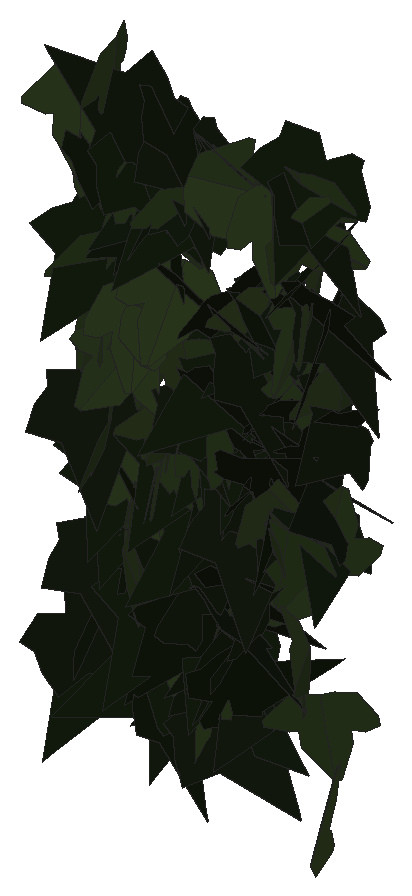
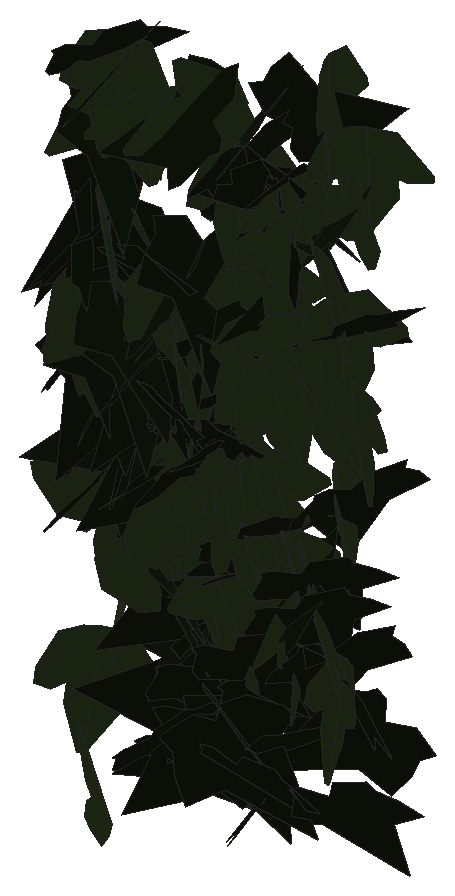
# SketchUp Ruby script. Lengths in inches.
U = 1.inch
M = Sketchup.active_model
def pt(a) = Geom::Point3d.new(a.map { |v| v * U })
def face(e, loops, mat)
  f = e.add_face(loops[0].map { |a| pt(a) })
  loops[1..].each { |l| e.add_face(l.map { |a| pt(a) }).erase! }
  f.material = f.back_material = mat if mat
  f
end
# faces: each face lists its corners as indices into pts; further lists are holes
def faces(e, pts, list, mat = nil) = list.each { |f| face(e, (f[0].is_a?(Array) ? f : [f]).map { |l| l.map { |i| pts[i] } }, mat) }
# xy, xz, yz: faces in a plane at the given z, y or x. An outline is a flat list of corners, or four numbers for a rectangle; further outlines are holes
def ring(l) = l.size == 4 ? [[l[0], l[1]], [l[2], l[1]], [l[2], l[3]], [l[0], l[3]]] : l.each_slice(2).to_a
def flat(e, list, mat, &to3) = list.each { |f| face(e, (f[0].is_a?(Array) ? f : [f]).map { |l| ring(l).map { |u, v| to3.(u, v) } }, mat) }
def xy(e, z, list, mat = nil) = flat(e, list, mat) { |x, y| [x, y, z] }
def xz(e, y, list, mat = nil) = flat(e, list, mat) { |x, z| [x, y, z] }
def yz(e, x, list, mat = nil) = flat(e, list, mat) { |y, z| [x, y, z] }
def lines(e, pts, list) = list.each { |a, b| e.add_line(pt(pts[a]), pt(pts[b])) }
# prism: a flat outline (further loops are holes) pulled along v
def prism(e, loops, v, mat = nil)
  f = face(e, loops, mat); d = Geom::Vector3d.new(v.map { |x| x * U })
  f.pushpull(f.normal.samedirection?(d) ? d.length : -d.length)
end
def box(e, o, s, mat = nil) = prism(e, [[o, [o[0] + s[0], o[1], o[2]], [o[0] + s[0], o[1] + s[1], o[2]], [o[0], o[1] + s[1], o[2]]]], [0, 0, s[2]], mat)
def at(x, y, z, deg = 0) = Geom::Transformation.translation(pt([x, y, z])) * Geom::Transformation.rotation(ORIGIN, Z_AXIS, deg.degrees)
def axes(o, x, y, z) = Geom::Transformation.new([*x, 0, *y, 0, *z, 0, *pt(o).to_a, 1])
def part(name) = M.definitions.add(name)
# library, detail: a bought-in or finely detailed component or shape, given as its bounding box
def library(name, o, s) = part(name).tap { |d| box(d.entities, o, s) }
def detail(e, o, s) = box(e.add_group.entities, o, s)
def put(e, d, t, mat = nil) = e.add_instance(d, t).tap { |i| i.material = mat if mat }
def group(e, t, mat = nil) = e.add_group.tap { |g| g.transformation = t; g.material = mat if mat }.entities
root = M.entities
M.materials.add("efeu1").color = [18, 25, 13]
M.materials.add("efeu2").color = [43, 57, 29]
c1 = part("ivyleaf_9")
p = [[1.54,2.16,1.25],[1.36,2.04,1.19],[-0.21,0.99,0.68],[-0.71,1.11,0.82],[-0.85,0.86,0.67],[-0.8,0.17,0.21],
  [-0.9,-0.01,0.1],[-0.67,-0.16,-0.02],[-0.08,-0.08,-0.05],[-0.03,-0.6,-0.4],[0.65,-0.88,-0.66],[0.83,-0.6,-0.49],
  [1.29,-0.42,-0.43],[1.8125,-0.07,-0.26],[1.21,0.44,0.15]]
faces(c1.entities,p,[[0,1,2,3,4,5,6,7,8,9,10,11,12,13,14]],"efeu1")
c2 = part("ivyleaf_10")
p = [[0,0.5,-0.03],[-0.0625,2.02,-0.43],[-0.19,2.01,-0.46],[-0.54,1.05,-0.29],[-0.52,0.625,-0.18],[-0.83,0.76,-0.28],
  [-1.16,0.64,-0.33],[-1.15,0.33,-0.24],[-0.77,-0.39,0.02],[-0.3,-0.51,0.16],[0.04,-0.48,0.23],[-0.02,2.01,-0.4375],
  [-0.06,2.01,-0.43],[0.04,-0.49,0.23],[0.67,-0.49,0.14],[1.38,0.36,-0.2],[1.375,0.51,-0.24],[0.81,0.65,-0.19],
  [0.62,0.59,-0.15],[0.6,1.09,-0.28],[0.5,1.23,-0.31]]
faces(c2.entities,p,[[0,1,2,3,4,5,6,7,8,9,10],[11,12,0,13,14,15,16,17,18,19,20]],"efeu2")
put(root,c1,axes([43.54,222.53,237.25],[0.46224,0.15127,-0.116],[0.11056,0.0351,0.48636],[0.15529,-0.47527,-0.00101]))
put(root,c1,axes([44.33,222.78,241.43],[-0.26887,-0.42118,0.01772],[0.03089,-0.04064,-0.49739],[0.42042,-0.26637,0.04787]))
put(root,c1,axes([41.21,222.68,237.46],[-0.08597,-0.48303,-0.09641],[0.03491,0.09165,-0.49029],[0.49131,-0.09104,0.01797]))
put(root,c1,axes([43.4,222.62,238.74],[0.20242,-0.4554,-0.0405],[-0.01543,0.03746,-0.49836],[0.45693,0.20301,0.00111]))
put(root,c2,axes([41.53,222.4375,237.27],[0.17347,-0.43056,-0.18582],[-0.06305,0.17491,-0.46415],[0.46469,0.18446,0.00639]))
put(root,c1,axes([42.93,222.35,235.55],[-0.116,0.12484,0.47006],[-0.34623,0.31818,-0.16994],[-0.34156,-0.36493,0.01263]))
put(root,c1,axes([42.04,222.5,241.2],[-0.05864,0.03305,0.49545],[-0.45265,0.20154,-0.06702],[-0.20414,-0.45639,0.00628]))
put(root,c2,axes([41.1,222.62,241.3],[-0.45326,-0.21028,0.0183],[0.06607,-0.18252,-0.46078],[0.20047,-0.4153,0.19324]))
put(root,c2,axes([41.92,222.54,238.97],[0.36604,0.3394,-0.02879],[-0.02117,-0.01951,-0.49917],[-0.33996,0.36665,0.00008]))
put(root,c2,axes([44.09,222.59,239.52],[0.39246,-0.30886,-0.02416],[-0.01952,0.01427,-0.49942],[0.30918,0.39294,-0.00086]))
put(root,c1,axes([42.7,222.65,235.28],[0.06829,0.23595,-0.43551],[-0.10368,-0.42308,-0.24547],[-0.48434,0.12384,-0.00886]))
put(root,c1,axes([43.36,222.73,236.66],[-0.10242,-0.48425,-0.07077],[0.02536,0.06696,-0.49485],[0.48874,-0.10495,0.01084]))
put(root,c1,axes([42.11,222.46,240.21],[-0.36634,0.33812,0.03838],[-0.0259,0.02852,-0.49851],[-0.3393,-0.36724,-0.00339]))
put(root,c2,axes([44,222.83,235.11],[-0.14747,0.00715,0.4777],[0.3485,-0.34037,0.11268],[0.32681,0.36619,0.09541]))
put(root,c1,axes([42.43,222.63,239.28],[0.27758,-0.26965,0.31661],[0.29438,-0.14148,-0.37859],[0.29376,0.39658,0.08022]))
put(root,c1,axes([44.24,222.6,241.11],[0.23225,-0.43216,-0.09644],[-0.01298,0.10221,-0.48927],[0.4426,0.22977,0.03625]))
put(root,c2,axes([41.75,222.55,238.27],[0.42519,0.0263,-0.26177],[-0.26303,0.05257,-0.42196],[0.00533,0.49653,0.05854]))
put(root,c2,axes([44.39,222.31,240.8125],[-0.19601,-0.26063,-0.37901],[0.24554,0.28909,-0.32578],[0.38896,-0.31384,0.01467]))
put(root,c2,axes([42.41,222.6,239.36],[0.41704,0.24252,-0.13138],[-0.12281,-0.04998,-0.4821],[-0.24697,0.43438,0.01788]))
put(root,c1,axes([42.53,222.83,240.49],[-0.38364,-0.30971,0.08308],[-0.06938,-0.04631,-0.49299],[0.31306,-0.38979,-0.00744]))
put(root,c1,axes([42.48,222.67,240.68],[-0.49563,0.05348,0.03861],[-0.03939,-0.0052,-0.49842],[-0.05291,-0.4971,0.00937]))
put(root,c1,axes([42.11,222.9,234.29],[-0.37796,-0.1692,0.28022],[-0.19084,-0.23386,-0.39861],[0.26595,-0.40827,0.1122]))
put(root,c1,axes([41.08,222.41,234.77],[0.07274,-0.12619,-0.47831],[0.24955,0.42679,-0.07464],[0.42712,-0.22787,0.12507]))
put(root,c1,axes([41.24,222.47,240.75],[0.37142,-0.27383,-0.19253],[-0.11361,0.16739,-0.45725],[0.31487,0.38341,0.06212]))
put(root,c2,axes([43.79,222.56,240.81],[0.25572,0.42952,-0.01094],[-0.00033,-0.01254,-0.49984],[-0.42966,0.25565,-0.00612]))
put(root,c2,axes([42.67,222.55,240.52],[-0.30459,-0.39138,-0.06357],[0.04452,0.04589,-0.49589],[0.39401,-0.30775,0.00689]))
put(root,c1,axes([41.21,222.94,239.34],[-0.28961,-0.38438,0.13557],[0.00723,-0.17112,-0.46975],[0.40752,-0.27013,0.10467]))
put(root,c2,axes([44.03,222.56,236.66],[-0.46662,-0.11221,0.14027],[-0.13807,-0.02574,-0.47987],[0.11492,-0.48657,-0.00697]))
put(root,c2,axes([41.53,222.58,241.92],[0.12375,-0.4795,-0.06904],[0.0585,0.08553,-0.48914],[0.4809,0.11299,0.07727]))
put(root,c2,axes([41.09,222.72,240.63],[0.22306,-0.06731,0.4424],[0.43464,-0.08499,-0.23208],[0.10644,0.4881,0.02059]))
put(root,c1,axes([42.25,222.77,241.34],[0.2103,-0.44999,0.05732],[0.0192,-0.0543,-0.49667],[0.45322,0.2111,-0.00556]))
put(root,c1,axes([43.06,222.78,237.04],[-0.45318,0.0002,-0.21125],[0.20958,-0.06218,-0.44968],[-0.02646,-0.49612,0.05628]))
put(root,c1,axes([42.84,222.71,237.83],[0.17704,-0.14553,0.44438],[0.36361,-0.25593,-0.22867],[0.29402,0.40413,0.01521]))
put(root,c1,axes([43.07,222.69,235.41],[0.32484,-0.3525,0.14222],[0.15011,-0.0529,-0.47399],[0.34921,0.35064,0.07146]))
put(root,c1,axes([41.84,222.59,240.82],[0.18669,-0.4129,-0.21134],[0.01255,0.23223,-0.44262],[0.46367,0.15996,0.09707]))
put(root,c2,axes([44.24,222.5625,241.21],[-0.49734,-0.05058,0.00982],[-0.01012,0.00247,-0.49989],[0.05052,-0.49743,-0.00349]))
put(root,c1,axes([41.35,222.76,235.65],[-0.09243,-0.45518,-0.18513],[0.06497,0.1754,-0.4637],[0.48707,-0.10978,0.02672]))
put(root,c1,axes([43.11,222.89,238.35],[-0.45024,-0.18225,0.11861],[-0.11115,-0.04152,-0.48572],[0.18689,-0.46375,-0.00313]))
put(root,c1,axes([44.48,222.375,240.3125],[-0.08007,0.47021,0.14998],[-0.06984,0.13962,-0.475],[-0.48858,-0.09701,0.04332]))
put(root,c1,axes([42.11,222.95,235.14],[-0.32486,-0.37401,0.0677],[-0.04828,-0.04773,-0.49537],[0.37701,-0.32839,-0.00511]))
put(root,c2,axes([41.95,222.61,240.55],[0.06822,0.49532,0.0024],[-0.00265,0.00279,-0.49999],[-0.49532,0.06821,0.00301]))
put(root,c2,axes([43.09,222.375,240.93],[0.11835,0.09672,0.47606],[0.23167,0.41944,-0.14282],[-0.42699,0.25438,0.05447]))
put(root,c1,axes([44.29,223.07,237.1],[-0.05895,-0.18464,0.46091],[-0.05296,-0.45916,-0.19071],[0.49368,-0.0713,0.03458]))
put(root,c2,axes([42.57,222.77,234.35],[0.4838,-0.09505,0.08308],[0.08028,-0.02229,-0.49301],[0.09743,0.49038,-0.00631]))
put(root,c1,axes([43.01,222.48,235.76],[0.46479,0.09077,0.16041],[0.1566,0.03504,-0.47355],[-0.09721,0.49044,0.00414]))
put(root,c1,axes([43.17,222.7,235.24],[-0.4087,0.28596,-0.03458],[0.03373,-0.0121,-0.49871],[-0.28606,-0.40998,-0.0094]))
put(root,c2,axes([41.88,222.5,235.68],[-0.2152,0.38535,0.23494],[-0.15893,0.1789,-0.43902],[-0.42241,-0.26363,0.04549]))
put(root,c1,axes([42.05,222.83,233.95],[0.23568,-0.44035,-0.02338],[-0.01161,0.02031,-0.49945],[0.44082,0.23597,-0.00065]))
put(root,c2,axes([43.89,222.55,237.2],[-0.21134,-0.35607,-0.28026],[0.14901,0.23744,-0.41403],[0.42794,-0.25852,0.00575]))
put(root,c1,axes([41.16,222.9,235.44],[-0.36905,-0.02771,-0.33621],[0.33735,-0.03036,-0.3678],[-0.00004,-0.49831,0.0411]))
put(root,c1,axes([42.37,222.875,241.01],[0.05277,-0.48849,-0.09269],[-0.01564,0.09153,-0.4913],[0.49696,0.05475,-0.00562]))
put(root,c1,axes([42.65,223.11,236.08],[-0.37114,-0.26984,0.1986],[-0.04136,-0.25721,-0.42677],[0.33249,-0.33321,0.1686]))
put(root,c1,axes([44.39,223.14,238.08],[-0.08884,-0.31186,0.38059],[-0.03628,-0.38154,-0.32111],[0.4907,-0.08467,0.04516]))
put(root,c1,axes([43.69,222.59,235.79],[-0.30283,0.36432,0.15988],[-0.11252,0.11429,-0.47358],[-0.38162,-0.32281,0.01276]))
put(root,c2,axes([42.15,222.46,238.94],[0.15593,0.16079,0.44703],[0.22157,0.39157,-0.21813],[-0.42023,0.26612,0.05087]))
put(root,c2,axes([42.5,222.71,238.44],[-0.4486,-0.21904,-0.02789],[0.02371,0.01499,-0.49921],[0.21953,-0.44922,-0.00306]))
put(root,c2,axes([43.61,222.59,236.78],[-0.36045,0.1622,0.30621],[-0.28549,0.1114,-0.39507],[-0.19639,-0.45965,0.01231]))
put(root,c2,axes([41.28,222.77,239.375],[-0.18752,-0.46324,-0.0158],[-0.0017,0.01773,-0.49968],[0.4635,-0.18734,-0.00822]))
put(root,c2,axes([42.05,222.91,238.5],[-0.13518,-0.45783,0.14871],[-0.02121,-0.14865,-0.47692],[0.48091,-0.13524,0.02077]))
put(root,c2,axes([41.48,222.8,239.94],[0.37888,-0.31492,-0.0853],[-0.05638,0.06556,-0.49247],[0.32136,0.38279,0.01417]))
put(root,c1,axes([42.95,222.77,241.05],[0.41235,-0.2487,0.13461],[0.15086,-0.00785,-0.47663],[0.23919,0.43369,0.06856]))
put(root,c1,axes([41.9,222.93,240.36],[-0.12662,-0.0082,-0.48363],[0.48362,0.00724,-0.12674],[0.00908,-0.49988,0.0061]))
put(root,c1,axes([44.03,222.625,239.7],[0.49536,0.04115,0.05411],[0.05474,-0.00553,-0.49696],[-0.0403,0.49827,-0.00998]))
put(root,c2,axes([41.8125,222.875,236.68],[0.38641,-0.31726,0.00575],[0.00385,-0.00438,-0.49997],[0.31728,0.38643,-0.00094]))
put(root,c2,axes([42.19,222.8125,237.06],[-0.41634,0.1016,0.25756],[-0.27576,-0.1106,-0.40215],[-0.02474,-0.47691,0.14813]))
put(root,c2,axes([41.08,222.77,238.52],[0.4018,-0.27518,-0.11329],[-0.04383,0.13354,-0.47984],[0.29434,0.39553,0.08319]))
put(root,c1,axes([43.15,222.61,239.49],[-0.02074,0.49729,-0.04769],[0.01255,-0.0472,-0.49761],[-0.49941,-0.02184,-0.01052]))
put(root,c1,axes([41.16,223.03,234.17],[-0.42793,-0.25439,-0.04647],[0.0371,0.02852,-0.49781],[0.25592,-0.4295,-0.00553]))
put(root,c2,axes([41.76,222.89,236.61],[0.36146,-0.34541,0.00585],[-0.00138,-0.00991,-0.4999],[0.34546,0.36137,-0.00812]))
put(root,c1,axes([43.07,222.51,234.4],[0.16173,0.08903,0.46467],[0.41569,0.20777,-0.18449],[-0.22594,0.44599,-0.00681]))
put(root,c1,axes([43.04,223.03,237.63],[-0.36746,-0.30638,-0.14526],[0.13957,0.05853,-0.47654],[0.30901,-0.39077,0.04251]))
put(root,c2,axes([43.9,222.93,235.93],[-0.1448,0.08012,-0.47182],[-0.47458,-0.08756,0.13078],[-0.06167,0.48571,0.1014]))
put(root,c2,axes([44.33,222.79,234.6],[-0.41247,-0.27968,-0.04056],[0.03592,0.01929,-0.49833],[0.28031,-0.41401,0.00417]))
put(root,c2,axes([44.28,222.8,232.89],[0.32162,-0.37822,0.05926],[-0.03848,0.04507,0.49648],[-0.3809,-0.32391,-0.00012]))
put(root,c1,axes([43.63,223.125,237.17],[-0.07854,0.04571,-0.49167],[0.38472,-0.30643,-0.08994],[-0.30955,-0.39244,0.01296]))
put(root,c1,axes([42.7,222.86,234.59],[-0.43942,0.23839,0.00924],[-0.00679,0.00686,-0.49991],[-0.23847,-0.43946,-0.00279]))
put(root,c1,axes([42.5,222.96,237.71],[0.08377,-0.47898,-0.11644],[0.09221,0.13125,-0.47357],[0.48423,0.05787,0.11033]))
put(root,c1,axes([43.73,223,239.28],[-0.49983,-0.0111,0.00716],[-0.00729,0.00605,-0.49991],[0.01101,-0.49984,-0.00621]))
put(root,c1,axes([44.24,223.13,239.47],[-0.19198,0.02738,-0.46086],[0.38663,-0.26324,-0.1767],[-0.25231,-0.42421,0.07991]))
put(root,c2,axes([44.28,222.9,236.47],[-0.40174,-0.28743,0.07738],[0.06544,0.04151,0.49396],[-0.29038,0.40701,0.00427]))
put(root,c2,axes([42.6,222.86,237.44],[0.04224,0.49346,-0.06865],[-0.01449,-0.06764,-0.49519],[-0.498,0.04383,0.00859]))
put(root,c2,axes([41.75,222.83,236.68],[0.47502,0.07575,0.13643],[0.11641,0.1191,-0.47145],[-0.10392,0.47966,0.09552]))
put(root,c1,axes([44.08,223.22,236.74],[-0.01739,-0.46494,0.1831],[0.0375,-0.18391,-0.46343],[0.49829,-0.00239,0.04127]))
put(root,c1,axes([42.83,222.85,233.99],[-0.00501,-0.28078,-0.41369],[0.24937,0.35717,-0.24544],[0.43335,-0.20879,0.13646]))
put(root,c2,axes([43.33,223.03,239.23],[-0.13587,-0.46833,0.11047],[-0.00946,-0.11217,-0.48716],[0.48109,-0.13447,0.02162]))
put(root,c2,axes([43.02,222.8,237.59],[0.00825,0.49162,0.0908],[-0.02455,0.09111,-0.49102],[-0.49933,0.00364,0.02564]))
put(root,c1,axes([42.71,223.17,235.14],[-0.29693,-0.39696,-0.06523],[0.03959,0.05184,-0.49573],[0.40033,-0.29956,0.00065]))
put(root,c2,axes([43.06,222.93,236.89],[-0.45518,-0.07823,-0.19156],[0.20073,-0.05458,-0.45468],[0.05023,-0.49082,0.08109]))
put(root,c1,axes([42.11,223.29,236.9],[-0.29805,-0.38784,0.10365],[0.01238,-0.13791,-0.48045],[0.40126,-0.28383,0.09181]))
put(root,c2,axes([42.11,223.03,237.4],[-0.23117,-0.43348,0.09303],[-0.03948,-0.08437,-0.49125],[0.44159,-0.23447,0.00478]))
put(root,c2,axes([43.23,222.86,238.66],[-0.43433,0.21175,0.12852],[-0.13258,0.0204,-0.48167],[-0.20923,-0.45249,0.03842]))
put(root,c2,axes([42.54,223.05,235.54],[0.44209,-0.20977,0.10271],[0.10163,-0.02519,-0.48891],[0.2103,0.45317,0.02036]))
put(root,c1,axes([44.16,222.63,237.95],[0.19586,0.44313,0.12358],[0.06323,0.10711,-0.48428],[-0.45568,0.20533,-0.01408]))
put(root,c1,axes([43.22,223.03,239.13],[0.34758,-0.35737,0.03839],[0.06158,0.00659,-0.49615],[0.35411,0.34964,0.04859]))
put(root,c2,axes([44.03,223.03,239.75],[0.29733,-0.40189,-0.00863],[0.03524,0.03675,-0.4974],[0.40044,0.29518,0.05018]))
put(root,c2,axes([44.39,222.98,238.72],[-0.05699,-0.49233,-0.06607],[0.01266,0.06504,-0.49559],[0.49658,-0.05816,0.00505]))
put(root,c2,axes([41.28,223.11,236.2],[0.36967,-0.32472,0.08886],[0.06679,-0.05861,-0.49204],[0.32997,0.37566,0.00005]))
put(root,c1,axes([44.23,223.07,239.43],[0.16513,-0.45771,-0.11504],[-0.001,0.12154,-0.485],[0.47194,0.16041,0.03922]))
put(root,c1,axes([42.64,222.93,234.22],[0.06672,-0.2029,-0.45209],[0.32479,0.36242,-0.11472],[0.37424,-0.27836,0.18016]))
put(root,c1,axes([44.02,222.78,238.35],[0.09409,0.48324,-0.08731],[-0.06881,-0.07505,-0.48952],[-0.48622,0.10414,0.05239]))
put(root,c2,axes([42.22,223.02,237.41],[0.06589,-0.4939,-0.04144],[0.01246,0.04345,-0.49795],[0.49548,0.06459,0.01803]))
put(root,c1,axes([43.58,222.9,237.46],[0.44155,-0.16585,0.16591],[0.19303,0.05591,-0.45784],[0.13332,0.46837,0.1134]))
put(root,c1,axes([42.93,223.22,237.71],[-0.45632,-0.20192,-0.03163],[0.02986,0.01068,-0.49899],[0.20218,-0.45729,0.00231]))
put(root,c1,axes([41.33,223.27,236.73],[-0.32225,-0.38019,-0.04017],[0.0591,0.00237,-0.49649],[0.37771,-0.32474,0.04341]))
put(root,c1,axes([43.36,223.15,238.4],[0.1694,-0.46954,-0.02898],[0.00779,0.0336,-0.49881],[0.47036,0.16855,0.0187]))
put(root,c1,axes([42.78,223.22,237.48],[0.00666,-0.49913,-0.02866],[0.01569,0.02885,-0.49892],[0.49971,0.00574,0.01605]))
put(root,c2,axes([43.11,223.34,236.84],[-0.21403,-0.26133,0.36864],[0.02211,-0.41347,-0.28027],[0.45133,-0.10367,0.18855]))
put(root,c2,axes([41.66,222.99,240.47],[0.04416,0.49717,-0.02958],[-0.00834,-0.02895,-0.49909],[-0.49798,0.04457,0.00574]))
put(root,c1,axes([42.51,223.125,234.56],[0.0416,0.17873,-0.46511],[-0.27166,-0.38312,-0.17152],[-0.4177,0.26697,0.06523]))
put(root,c2,axes([41.19,222.9375,235.42],[-0.42153,0.24684,0.1067],[-0.10347,0.03425,-0.48798],[-0.24821,-0.43347,0.02221]))
put(root,c1,axes([42.17,223.25,234.27],[-0.42098,-0.18976,-0.19174],[0.1982,0.0235,-0.45844],[0.183,-0.46199,0.05543]))
put(root,c1,axes([41.4,223.04,236.49],[0.40616,-0.28758,-0.04832],[-0.03482,0.03443,-0.4976],[0.28952,0.40757,0.00794]))
put(root,c2,axes([44.09,223.1,238.58],[-0.30165,-0.39719,0.03529],[0.01537,-0.05579,-0.49664],[0.39846,-0.29854,0.04587]))
put(root,c2,axes([41.62,223.1,236.2],[-0.06918,0.47547,-0.13836],[-0.02671,-0.14308,-0.47835],[-0.49447,-0.0588,0.0452]))
put(root,c1,axes([43.45,223.42,236.99],[-0.11328,-0.44687,0.19358],[0.00571,-0.19995,-0.45824],[0.48696,-0.10161,0.05041]))
put(root,c1,axes([43.09,223.44,234.37],[-0.20632,-0.41721,0.18267],[-0.00871,-0.19689,-0.45952],[0.45536,-0.1928,0.07398]))
put(root,c1,axes([41.34,223.36,236.375],[-0.28498,-0.40965,-0.03119],[0.05013,0.00299,-0.49747],[0.40777,-0.28667,0.03937]))
put(root,c2,axes([42.42,223.16,236.1],[0.46056,0.16249,-0.10713],[-0.10304,-0.02989,-0.48835],[-0.16511,0.47191,0.00596]))
put(root,c2,axes([42.96,223.16,238.42],[0.35293,-0.35214,0.03798],[0.07583,0.02275,-0.49369],[0.34596,0.35424,0.06947]))
put(root,c1,axes([42.1,223.36,235.63],[-0.38823,-0.31418,-0.02387],[0.02319,0.00928,-0.49938],[0.31423,-0.38885,0.00737]))
put(root,c1,axes([43.24,222.96,238.39],[0.48936,0.06616,-0.07841],[-0.07651,-0.01929,-0.49374],[-0.06836,0.49523,-0.00875]))
put(root,c1,axes([43.33,223.24,237.99],[-0.49633,0.05318,-0.02883],[0.03006,0.01007,-0.49899],[-0.05249,-0.49706,-0.01319]))
put(root,c1,axes([43.43,222.71,237.08],[0.19191,0.30901,0.34305],[0.14335,0.31326,-0.36238],[-0.43889,0.23744,0.03164]))
put(root,c1,axes([43.75,222.87,238.36],[-0.08661,0.48097,0.10568],[-0.02133,0.10354,-0.4887],[-0.49198,-0.08916,0.00258]))
put(root,c2,axes([42.17,223.26,237.13],[-0.0223,-0.48899,0.10192],[0.02282,-0.10291,-0.48876],[0.49898,-0.01715,0.02691]))
put(root,c1,axes([43.78,222.94,238.71],[-0.08088,0.4933,0.01047],[-0.11617,-0.00873,-0.48624],[-0.47954,-0.08109,0.11603]))
